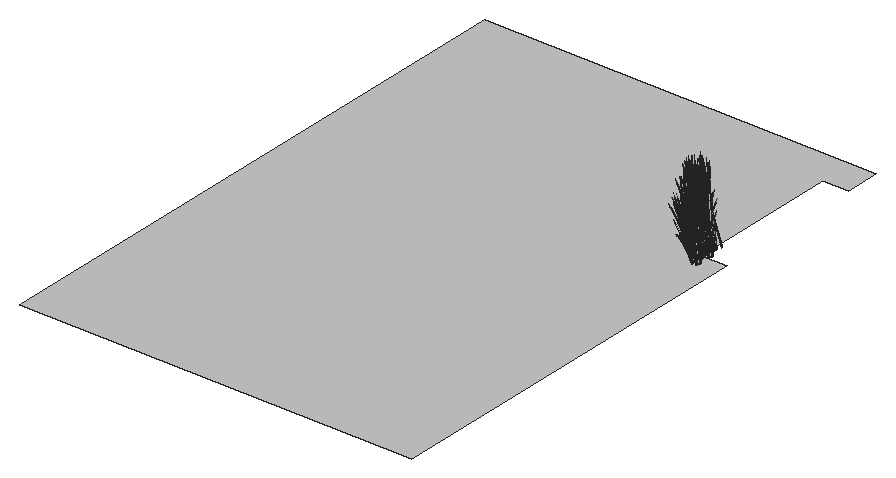
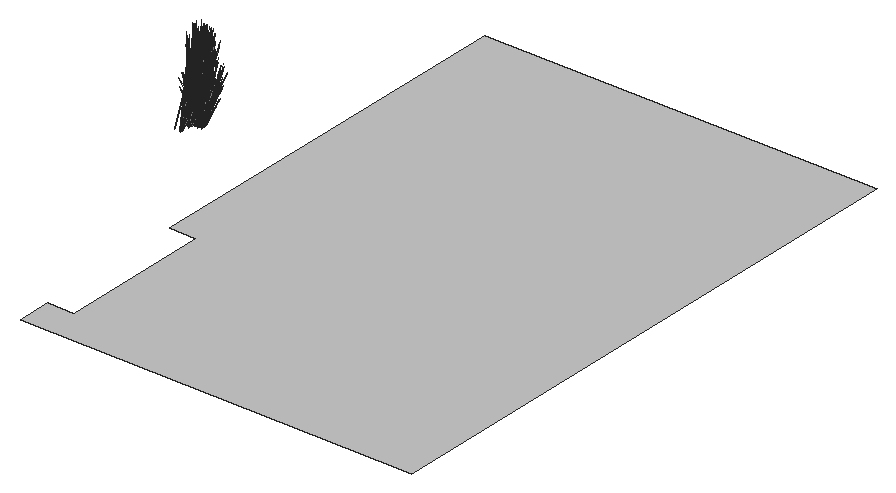
# SketchUp Ruby script. Lengths in inches.
U = 1.inch
M = Sketchup.active_model
def pt(a) = Geom::Point3d.new(a.map { |v| v * U })
def face(e, loops, mat)
  f = e.add_face(loops[0].map { |a| pt(a) })
  loops[1..].each { |l| e.add_face(l.map { |a| pt(a) }).erase! }
  f.material = f.back_material = mat if mat
  f
end
# faces: each face lists its corners as indices into pts; further lists are holes
def faces(e, pts, list, mat = nil) = list.each { |f| face(e, (f[0].is_a?(Array) ? f : [f]).map { |l| l.map { |i| pts[i] } }, mat) }
# xy, xz, yz: faces in a plane at the given z, y or x. An outline is a flat list of corners, or four numbers for a rectangle; further outlines are holes
def ring(l) = l.size == 4 ? [[l[0], l[1]], [l[2], l[1]], [l[2], l[3]], [l[0], l[3]]] : l.each_slice(2).to_a
def flat(e, list, mat, &to3) = list.each { |f| face(e, (f[0].is_a?(Array) ? f : [f]).map { |l| ring(l).map { |u, v| to3.(u, v) } }, mat) }
def xy(e, z, list, mat = nil) = flat(e, list, mat) { |x, y| [x, y, z] }
def xz(e, y, list, mat = nil) = flat(e, list, mat) { |x, z| [x, y, z] }
def yz(e, x, list, mat = nil) = flat(e, list, mat) { |y, z| [x, y, z] }
def lines(e, pts, list) = list.each { |a, b| e.add_line(pt(pts[a]), pt(pts[b])) }
# prism: a flat outline (further loops are holes) pulled along v
def prism(e, loops, v, mat = nil)
  f = face(e, loops, mat); d = Geom::Vector3d.new(v.map { |x| x * U })
  f.pushpull(f.normal.samedirection?(d) ? d.length : -d.length)
end
def box(e, o, s, mat = nil) = prism(e, [[o, [o[0] + s[0], o[1], o[2]], [o[0] + s[0], o[1] + s[1], o[2]], [o[0], o[1] + s[1], o[2]]]], [0, 0, s[2]], mat)
def at(x, y, z, deg = 0) = Geom::Transformation.translation(pt([x, y, z])) * Geom::Transformation.rotation(ORIGIN, Z_AXIS, deg.degrees)
def axes(o, x, y, z) = Geom::Transformation.new([*x, 0, *y, 0, *z, 0, *pt(o).to_a, 1])
def part(name) = M.definitions.add(name)
# library, detail: a bought-in or finely detailed component or shape, given as its bounding box
def library(name, o, s) = part(name).tap { |d| box(d.entities, o, s) }
def detail(e, o, s) = box(e.add_group.entities, o, s)
def put(e, d, t, mat = nil) = e.add_instance(d, t).tap { |i| i.material = mat if mat }
def group(e, t, mat = nil) = e.add_group.tap { |g| g.transformation = t; g.material = mat if mat }.entities
root = M.entities
M.materials.add("LightPink_Translucent").color = [144, 107, 117]
M.materials["LightPink_Translucent"].alpha = 0.75
M.materials.add("[_0053_Ivory_]").color = [200, 200, 200]
c1 = part("blade")
p = [[2.15,0.21,22],[0,0.17,0],[0.09,0.45,0],[2.18,0.31,22],[2.29,0.31,22],[0.38,0.45,0],
  [2.48,0.24,33],[2.49,0.24,33],[2.48,0.22,33]]
faces(c1.entities,p,[[0,1,2,3],[4,5,2,3],[6,3,4,7],[8,0,3,6]])
c2 = part("seeds")
p = [[0.3,-0.1,1.38],[-0.01,-0.03,1.59],[-0.01,-0.03,0.03],[0.14,-0.07,-0.07],[0.29,-0.03,3],[0.15,0.01,3.11]]
faces(c2.entities,p,[[0,1,2,3],[1,0,4,5]],"LightPink_Translucent")
c3 = part("blade with seeds")
put(c3.entities,c1,at(0,0,0))
put(c3.entities,c2,axes([2.4,0.25,30.99],[1.5799,-0.05474,1.17369],[-0.12525,1.92788,0.29478],[-0.07173,-0.02425,1.56792]))
xy(root,0,[[377.51,94.15,377.51,503.15,653.51,503.15,653.51,479.15,635.1,479.15,635.1,371.15,653.51,371.15,653.51,94.15]],"[_0053_Ivory_]")
put(root,c3,axes([670.81,318.54,37.53],[0.25192,-0.01424,1.71376],[-0.16712,0.61729,0.13857],[-0.35901,-0.03818,0.73262]),"[_0053_Ivory_]")
put(root,c3,axes([670.91,319.625,37.53],[0.21074,-0.13302,1.71376],[0.17741,0.61464,0.13857],[-0.33083,0.13891,0.73262]),"[_0053_Ivory_]")
put(root,c3,axes([670.25,320.67,36.24],[0.21107,0.05162,1.43002],[0.13604,0.52729,-0.30754],[-0.28671,0.0987,0.61141]),"[_0053_Ivory_]")
put(root,c3,axes([672.12,318.99,37],[0.17264,-0.09097,1.77064],[0.05953,0.63516,0.13857],[-0.37394,0.08428,0.63284]),"[_0053_Ivory_]")
put(root,c3,axes([671.56,317.97,38.63],[-0.60713,-0.01514,-0.71045],[0.04078,-0.63759,0.08574],[-0.25721,-0.06729,1.00501]),"[_0053_Ivory_]")
put(root,c3,axes([671.07,318.12,36.24],[0.11858,0.17508,1.43002],[-0.27325,0.4759,-0.30754],[-0.28057,-0.11375,0.61141]),"[_0053_Ivory_]")
put(root,c3,axes([670.58,319.07,38.18],[-0.50475,-0.17543,-0.35414],[0.14722,-0.5118,0.4572],[-0.20322,0.04693,0.87481]),"[_0053_Ivory_]")
put(root,c3,axes([671.28,317.55,37.53],[0.2256,0.10835,1.71376],[-0.46687,0.45453,0.13857],[-0.29098,-0.20505,0.73262]),"[_0053_Ivory_]")
put(root,c3,axes([670.93,319.33,38.33],[-0.16454,0.57202,-0.51099],[-0.56413,-0.19607,-0.3958],[-0.22713,0.05245,0.97773]),"[_0053_Ivory_]")
put(root,c3,axes([671.36,318.1,38.33],[-0.44101,0.41656,-0.51099],[-0.38623,-0.44004,-0.3958],[-0.22407,-0.06338,0.97773]),"[_0053_Ivory_]")
put(root,c3,axes([670.65,319.3,35.15],[0.0154,0.09911,1.76342],[-0.31051,0.51756,-0.26939],[-0.22056,-0.02609,0.30037]),"[_0053_Ivory_]")
put(root,c3,axes([669.8125,321.78,36.42],[0.25312,-0.28501,1.1486],[0.09988,0.45119,0.84392],[-0.18292,0.08079,0.25299]),"[_0053_Ivory_]")
put(root,c3,axes([671.19,317.7,38.18],[-0.34557,-0.39372,-0.35414],[0.39459,-0.37271,0.4572],[-0.20048,-0.05671,0.87481]),"[_0053_Ivory_]")
put(root,c3,axes([671.68,320.04,37.53],[0.1517,-0.19322,1.71376],[0.38303,0.52154,0.13857],[-0.26271,0.23751,0.73262]),"[_0053_Ivory_]")
put(root,c3,axes([670.77,320.55,38.18],[-0.52868,0.08987,-0.35414],[-0.1396,-0.51376,0.4572],[-0.1515,0.13799,0.87481]),"[_0053_Ivory_]")
put(root,c3,axes([670.48,322.07,35.15],[0.08147,0.06283,1.76342],[0.13814,0.58211,-0.26939],[-0.18056,0.12413,0.30037]),"[_0053_Ivory_]")
put(root,c3,axes([670.36,318.65,36.42],[0.38775,-0.045,1.1486],[-0.24596,0.39648,0.84392],[-0.19161,-0.05948,0.25299]),"[_0053_Ivory_]")
put(root,c3,axes([671.57,320.52,37.53],[0.11309,-0.21615,1.71376],[0.47441,0.44731,0.13857],[-0.21402,0.27879,0.73262]),"[_0053_Ivory_]")
put(root,c3,axes([671.2,320.61,38.33],[0.15602,0.5742,-0.51099],[-0.59087,0.10045,-0.3958],[-0.16933,0.15423,0.97773]),"[_0053_Ivory_]")
put(root,c3,axes([672.68,320.19,35.71],[-0.63179,-0.1031,-0.62353],[0.13332,-0.63596,-0.16365],[-0.18854,-0.07706,1.37633]),"[_0053_Ivory_]")
put(root,c3,axes([672.61,317.22,38.63],[-0.51789,-0.30395,-0.71045],[0.36805,-0.53263,0.08574],[-0.18764,-0.18149,1.00501]),"[_0053_Ivory_]")
put(root,c3,axes([672.37,317.23,38.33],[-0.59932,0.14948,-0.51099],[-0.10484,-0.56611,-0.3958],[-0.16097,-0.16223,0.97773]),"[_0053_Ivory_]")
put(root,c3,axes([671.85,321.4,35.67],[-0.56842,-0.31443,-0.49651],[0.33976,-0.56381,0],[-0.12946,-0.07161,1.57504]),"[_0053_Ivory_]")
put(root,c3,axes([671.6,316.71,35.15],[-0.05883,0.08284,1.76342],[-0.59454,0.17861,-0.26939],[-0.14363,-0.16248,0.30037]),"[_0053_Ivory_]")
put(root,c3,axes([672.19,321.78,36.03],[-0.37973,0.63014,0],[-0.6353,-0.35142,-0.51607],[-0.14469,-0.08004,1.63711]),"[_0053_Ivory_]")
put(root,c3,axes([671.5,322.69,36.24],[0.19166,-0.0992,1.43002],[0.4732,0.29912,-0.30754],[-0.14084,0.25882,0.61141]),"[_0053_Ivory_]")
put(root,c3,axes([671.23,317.03,35.78],[-0.1752,0.51349,-0.03893],[-0.53924,-0.15795,-0.17649],[-0.08187,-0.08399,0.58215]),"[_0053_Ivory_]")
put(root,c3,axes([672.03,316.39,36.24],[-0.03678,0.20572,1.43002],[-0.53767,0.17221,-0.30754],[-0.12568,-0.26589,0.61141]),"[_0053_Ivory_]")
put(root,c3,axes([672.21,316.92,37.53],[0.13883,0.2019,1.71376],[-0.64153,0.16998,0.13857],[-0.14499,-0.31697,0.73262]),"[_0053_Ivory_]")
put(root,c3,axes([673.39,320.29,36.32],[-0.61322,0.4175,-0.29095],[-0.40778,-0.58992,-0.50002],[-0.1513,-0.05991,1.59708]),"[_0053_Ivory_]")
put(root,c3,axes([672.43,316.8125,38.18],[-0.0938,-0.50652,-0.35414],[0.53623,-0.13375,0.4572],[-0.14403,-0.14515,0.87481]),"[_0053_Ivory_]")
put(root,c3,axes([670.94,319.38,36.03],[-0.75945,0,0],[0,-0.70283,-0.51607],[0,-0.16007,1.63711]),"[_0053_Ivory_]")
put(root,c3,axes([672.01,321.16,35.68],[-0.14267,-0.54795,-0.30978],[0.56663,-0.1556,0.30978],[-0.11423,-0.06319,1.38974]),"[_0053_Ivory_]")
put(root,c3,axes([671.7,321.74,38.18],[-0.41095,0.33109,-0.35414],[-0.38901,-0.37805,0.4572],[-0.05919,0.19208,0.87481]),"[_0053_Ivory_]")
put(root,c3,axes([673.8,320.74,35.71],[-0.40909,0.47266,-0.62353],[-0.50819,-0.4286,-0.16365],[-0.16393,0.11791,1.37633]),"[_0053_Ivory_]")
put(root,c3,axes([671.53,319.19,35.98],[-0.56493,0.5287,0.30756],[-0.56528,-0.52313,-0.36492],[-0.01973,-0.15014,1.64885]),"[_0053_Ivory_]")
put(root,c3,axes([673.85,320.65,36.98],[0.52485,0.25358,1.51261],[-0.51417,0.54629,0.59816],[-0.23031,-0.32378,1.26806]),"[_0053_Ivory_]")
put(root,c3,axes([671.85,316.06,36.42],[0.31682,0.21887,1.1486],[-0.4614,0.13157,0.84392],[-0.09872,-0.16821,0.25299]),"[_0053_Ivory_]")
put(root,c3,axes([674.08,320.48,36.12],[-0.59306,-0.50614,-0.25192],[0.49904,-0.56836,0.5513],[-0.1597,0.05921,1.68216]),"[_0053_Ivory_]")
put(root,c3,axes([673,319.99,35.86],[-0.36485,-0.52782,-0.44739],[0.55265,-0.37168,0.21531],[-0.11807,-0.06531,1.43643]),"[_0053_Ivory_]")
put(root,c3,axes([671.97,321.39,38.99],[-0.0158,0.58168,-0.7886],[-0.66548,-0.03907,0.09517],[-0.07023,0.24643,1.11556]),"[_0053_Ivory_]")
put(root,c3,axes([671.96,323.02,36.42],[-0.01572,-0.37392,1.1486],[0.39276,0.26669,0.84392],[-0.07724,0.17822,0.25299]),"[_0053_Ivory_]")
put(root,c3,axes([673.78,320.37,35.86],[-0.65953,0.03882,-0.44739],[-0.05964,-0.64439,0.21531],[-0.11807,0.06531,1.43643]),"[_0053_Ivory_]")
put(root,c3,axes([677.08,321.61,37.53],[0.25192,-0.01424,1.71376],[-0.16712,0.61729,0.13857],[-0.35901,-0.03818,0.73262]),"[_0053_Ivory_]")
put(root,c3,axes([672.52,321.45,36.13],[0.56842,0.31443,0.49651],[-0.33976,0.56381,0],[-0.12946,-0.07161,1.57504]),"[_0053_Ivory_]")
put(root,c3,axes([671.75,322.21,37.02],[0.01334,-0.32463,1.54345],[0.60018,0.17147,0.21329],[-0.052,0.34598,0.72882]),"[_0053_Ivory_]")
put(root,c3,axes([673.06,320.3,36.09],[0.16098,-0.74515,-0.23429],[0.76326,0.12989,0.51271],[-0.13337,-0.1029,1.5644]),"[_0053_Ivory_]")
put(root,c3,axes([673.34,320.47,36.27],[-0.11717,0.56122,0.1448],[-0.57245,-0.09742,-0.41347],[-0.10418,-0.05763,1.26744]),"[_0053_Ivory_]")
put(root,c3,axes([674.47,322.03,35.67],[-0.56842,0.31443,-0.49651],[-0.33976,-0.56381,0],[-0.12946,0.07161,1.57504]),"[_0053_Ivory_]")
put(root,c3,axes([671.11,318.9,35.67],[0,-0.62885,-0.49651],[0.67951,0,0],[0,-0.14322,1.57504]),"[_0053_Ivory_]")
put(root,c3,axes([671.4,319.48,36.13],[0,0.62885,0.49651],[-0.67951,0,0],[0,-0.14322,1.57504]),"[_0053_Ivory_]")
put(root,c3,axes([674.51,321.87,35.85],[-0.37499,-0.63235,-0.05142],[0.6353,-0.35142,0.51607],[-0.15655,0.0602,1.6363]),"[_0053_Ivory_]")
put(root,c3,axes([672.11,321.58,38.66],[0.43478,0.42253,-0.5672],[-0.45929,0.37004,-0.43934],[-0.06615,0.21468,1.08528]),"[_0053_Ivory_]")
put(root,c3,axes([674.34,321.79,35.68],[-0.56663,-0.1556,-0.30978],[0.14267,-0.54795,0.30978],[-0.11423,0.06319,1.38974]),"[_0053_Ivory_]")
put(root,c3,axes([677.1875,312.1,37.53],[0.21074,-0.13302,1.71376],[0.17741,0.61464,0.13857],[-0.33083,0.13891,0.73262]),"[_0053_Ivory_]")
put(root,c3,axes([677.1875,322.69,37.53],[0.21074,-0.13302,1.71376],[0.17741,0.61464,0.13857],[-0.33083,0.13891,0.73262]),"[_0053_Ivory_]")
put(root,c3,axes([672.89,319.63,36.32],[-0.68399,-0.30005,-0.29095],[0.32934,-0.63331,-0.50002],[-0.0215,-0.15549,1.59708]),"[_0053_Ivory_]")
put(root,c3,axes([674.67,319.44,36.5],[-0.01659,-0.59209,1.41272],[0.75089,0.15348,0.59816],[-0.1776,0.32398,1.3335]),"[_0053_Ivory_]")
put(root,c3,axes([676.53,313.15,36.24],[0.21107,0.05162,1.43002],[0.13604,0.52729,-0.30754],[-0.28671,0.0987,0.61141]),"[_0053_Ivory_]")
put(root,c3,axes([676.53,323.74,36.24],[0.21107,0.05162,1.43002],[0.13604,0.52729,-0.30754],[-0.28671,0.0987,0.61141]),"[_0053_Ivory_]")
put(root,c3,axes([671.63,322.21,36.48],[0.55175,-0.11136,0.06507],[0.12684,0.44864,-0.86304],[-0.03498,0.22711,0.7736]),"[_0053_Ivory_]")
put(root,c3,axes([674.24,320.2,36.32],[0.07077,0.71755,-0.29095],[-0.73712,0.04339,-0.50002],[-0.1298,0.09558,1.59708]),"[_0053_Ivory_]")
put(root,c3,axes([672.58,318.99,35.75],[-0.24943,-0.64486,-0.69835],[0.71849,-0.23224,-0.18329],[-0.02757,-0.21836,1.54149]),"[_0053_Ivory_]")
put(root,c3,axes([678.4,311.46,37],[0.17264,-0.09097,1.77064],[0.05953,0.63516,0.13857],[-0.37394,0.08428,0.63284]),"[_0053_Ivory_]")
put(root,c3,axes([678.4,322.05,37],[0.17264,-0.09097,1.77064],[0.05953,0.63516,0.13857],[-0.37394,0.08428,0.63284]),"[_0053_Ivory_]")
put(root,c3,axes([673.7,316.97,38.33],[-0.59704,-0.15764,-0.51099],[0.20464,-0.54049,-0.3958],[-0.05475,-0.21761,0.97773]),"[_0053_Ivory_]")
put(root,c3,axes([672.6,320.97,37.53],[-0.01487,-0.24136,1.71376],[0.64429,0.16012,0.13857],[-0.03985,0.34396,0.73262]),"[_0053_Ivory_]")
put(root,c3,axes([671.4,318.91,35.68],[0.42396,-0.39235,-0.30978],[0.42396,0.39235,0.30978],[0,-0.12637,1.38974]),"[_0053_Ivory_]")
put(root,c3,axes([673.32,316.38,35.78],[-0.4197,0.36076,-0.03893],[-0.38456,-0.39511,-0.17649],[-0.02707,-0.11196,0.58215]),"[_0053_Ivory_]")
put(root,c3,axes([673.15,319.9375,36.01],[0.76764,0.13249,0.45755],[-0.15622,0.74829,0.17955],[-0.11218,-0.07226,1.58856]),"[_0053_Ivory_]")
put(root,c3,axes([677.83,321.03,38.63],[-0.60713,-0.01514,-0.71045],[0.04078,-0.63759,0.08574],[-0.25721,-0.06729,1.00501]),"[_0053_Ivory_]")
put(root,c3,axes([677.35,321.19,36.24],[0.11858,0.17508,1.43002],[-0.27325,0.4759,-0.30754],[-0.28057,-0.11375,0.61141]),"[_0053_Ivory_]")
put(root,c3,axes([672.95,319.8,36.37],[-0.29468,0.56664,0.44739],[-0.61229,-0.27271,-0.21531],[0,-0.13062,1.43643]),"[_0053_Ivory_]")
put(root,c3,axes([673.92,317.07,38.63],[-0.28988,-0.51132,-0.71045],[0.59671,-0.28496,0.08574],[-0.06778,-0.24706,1.00501]),"[_0053_Ivory_]")
put(root,c3,axes([676.86,311.55,38.18],[-0.50475,-0.17543,-0.35414],[0.14722,-0.5118,0.4572],[-0.20322,0.04693,0.87481]),"[_0053_Ivory_]")
put(root,c3,axes([676.86,322.14,38.18],[-0.50475,-0.17543,-0.35414],[0.14722,-0.5118,0.4572],[-0.20322,0.04693,0.87481]),"[_0053_Ivory_]")
put(root,c3,axes([677.56,320.62,37.53],[0.2256,0.10835,1.71376],[-0.46687,0.45453,0.13857],[-0.29098,-0.20505,0.73262]),"[_0053_Ivory_]")
put(root,c3,axes([677.56,330.76,37.53],[0.2256,0.10835,1.71376],[-0.46687,0.45453,0.13857],[-0.29098,-0.20505,0.73262]),"[_0053_Ivory_]")
put(root,c3,axes([672.73,321.13,36.13],[0.65264,-0.16691,0.17642],[0.16115,0.62115,0.35086],[-0.05821,-0.0905,1.60407]),"[_0053_Ivory_]")
put(root,c3,axes([677.21,311.81,38.33],[-0.16454,0.57202,-0.51099],[-0.56413,-0.19607,-0.3958],[-0.22713,0.05245,0.97773]),"[_0053_Ivory_]")
put(root,c3,axes([677.21,322.4,38.33],[-0.16454,0.57202,-0.51099],[-0.56413,-0.19607,-0.3958],[-0.22713,0.05245,0.97773]),"[_0053_Ivory_]")
put(root,c3,axes([673.57,321.23,35.85],[-0.61229,-0.28233,0],[0.29468,-0.58663,0],[0,0,1.62707]),"[_0053_Ivory_]")
put(root,c3,axes([674.99,321.9375,36.03],[0.37973,0.63014,0],[-0.6353,0.35142,-0.51607],[-0.14469,0.08004,1.63711]),"[_0053_Ivory_]")
put(root,c3,axes([677.63,321.16,38.33],[-0.44101,0.41656,-0.51099],[-0.38623,-0.44004,-0.3958],[-0.22407,-0.06338,0.97773]),"[_0053_Ivory_]")
put(root,c3,axes([676.92,311.77,35.15],[0.0154,0.09911,1.76342],[-0.31051,0.51756,-0.26939],[-0.22056,-0.02609,0.30037]),"[_0053_Ivory_]")
put(root,c3,axes([676.92,322.36,35.15],[0.0154,0.09911,1.76342],[-0.31051,0.51756,-0.26939],[-0.22056,-0.02609,0.30037]),"[_0053_Ivory_]")
put(root,c3,axes([674.68,321.17,36.13],[0.17545,-0.62497,0.17642],[0.64204,0.17686,0.35086],[-0.11091,0.00304,1.60407]),"[_0053_Ivory_]")
put(root,c3,axes([674.38,320.34,36.27],[0.44871,0.37783,0.1448],[-0.37428,0.42627,-0.41347],[-0.10418,0.05763,1.26744]),"[_0053_Ivory_]")
put(root,c3,axes([676.09,314.25,36.42],[0.25312,-0.28501,1.1486],[0.09988,0.45119,0.84392],[-0.18292,0.08079,0.25299]),"[_0053_Ivory_]")
put(root,c3,axes([676.09,324.85,36.42],[0.25312,-0.28501,1.1486],[0.09988,0.45119,0.84392],[-0.18292,0.08079,0.25299]),"[_0053_Ivory_]")
put(root,c3,axes([674.22,319.87,35.95],[-0.56493,-0.54126,-0.06131],[0.56528,-0.54159,0],[-0.01973,-0.0189,1.75571]),"[_0053_Ivory_]")
put(root,c3,axes([674.37,320.06,36.37],[0.65953,-0.03882,0.44739],[0.05964,0.64439,-0.21531],[-0.11807,0.06531,1.43643]),"[_0053_Ivory_]")
put(root,c3,axes([674.53,321.54,35.98],[0.76036,0.2044,0.30756],[-0.19023,0.7306,-0.36492],[-0.12585,0.09144,1.64885]),"[_0053_Ivory_]")
put(root,c3,axes([673.42,315.9375,35.15],[-0.10187,0.02266,1.76342],[-0.56336,-0.25503,-0.26939],[0.00945,-0.21273,0.30037]),"[_0053_Ivory_]")
put(root,c3,axes([674.86,321.5,36.13],[0.56842,-0.31443,0.49651],[0.33976,0.56381,0],[-0.12946,0.07161,1.57504]),"[_0053_Ivory_]")
put(root,c3,axes([677.47,320.77,38.18],[-0.34557,-0.39372,-0.35414],[0.39459,-0.37271,0.4572],[-0.20048,-0.05671,0.87481]),"[_0053_Ivory_]")
put(root,c3,axes([677.47,330.91,38.18],[-0.34557,-0.39372,-0.35414],[0.39459,-0.37271,0.4572],[-0.20048,-0.05671,0.87481]),"[_0053_Ivory_]")
put(root,c3,axes([673.98,316.64,38.18],[0.1831,-0.48359,-0.35414],[0.53419,0.14105,0.4572],[-0.04898,-0.1947,0.87481]),"[_0053_Ivory_]")
put(root,c3,axes([673.08,319.25,36.01],[0.26406,0.70318,0.45755],[-0.7545,0.24452,0.17955],[0.00922,-0.12921,1.58856]),"[_0053_Ivory_]")
put(root,c3,axes([677.96,312.52,37.53],[0.1517,-0.19322,1.71376],[0.38303,0.52154,0.13857],[-0.26271,0.23751,0.73262]),"[_0053_Ivory_]")
put(root,c3,axes([677.96,323.11,37.53],[0.1517,-0.19322,1.71376],[0.38303,0.52154,0.13857],[-0.26271,0.23751,0.73262]),"[_0053_Ivory_]")
put(root,c3,axes([677.04,313.02,38.18],[-0.52868,0.08987,-0.35414],[-0.1396,-0.51376,0.4572],[-0.1515,0.13799,0.87481]),"[_0053_Ivory_]")
put(root,c3,axes([677.04,323.61,38.18],[-0.52868,0.08987,-0.35414],[-0.1396,-0.51376,0.4572],[-0.1515,0.13799,0.87481]),"[_0053_Ivory_]")
put(root,c3,axes([672.96,319.16,35.86],[0.29468,-0.56664,-0.44739],[0.61229,0.27271,0.21531],[0,-0.13062,1.43643]),"[_0053_Ivory_]")
put(root,c3,axes([673.71,320.98,35.86],[-0.19817,-0.54216,0],[0.56587,-0.18986,0],[0,0,1.54371]),"[_0053_Ivory_]")
put(root,c3,axes([672.99,322.13,35.15],[0.09829,-0.03422,1.76342],[0.59126,0.18834,-0.26939],[0.01729,0.21228,0.30037]),"[_0053_Ivory_]")
put(root,c3,axes([676.76,314.55,35.15],[0.08147,0.06283,1.76342],[0.13814,0.58211,-0.26939],[-0.18056,0.12413,0.30037]),"[_0053_Ivory_]")
put(root,c3,axes([676.76,325.14,35.15],[0.08147,0.06283,1.76342],[0.13814,0.58211,-0.26939],[-0.18056,0.12413,0.30037]),"[_0053_Ivory_]")
put(root,c3,axes([673.125,322.32,38.18],[-0.1831,0.48359,-0.35414],[-0.53419,-0.14105,0.4572],[0.04898,0.1947,0.87481]),"[_0053_Ivory_]")
put(root,c3,axes([676.64,321.72,36.42],[0.38775,-0.045,1.1486],[-0.24596,0.39648,0.84392],[-0.19161,-0.05948,0.25299]),"[_0053_Ivory_]")
put(root,c3,axes([674.51,319.92,35.86],[-0.29468,0.56664,-0.44739],[-0.61229,-0.27271,0.21531],[0,0.13062,1.43643]),"[_0053_Ivory_]")
put(root,c3,axes([675.68,319.57,36.13],[-0.47719,-0.45806,0.17642],[0.48088,-0.44429,0.35086],[-0.0527,0.09355,1.60407]),"[_0053_Ivory_]")
put(root,c3,axes([674.03,319.31,35.86],[0,-0.72763,0],[0.75945,0,0],[0,0,1.79456]),"[_0053_Ivory_]")
put(root,c3,axes([677.84,312.99,37.53],[0.11309,-0.21615,1.71376],[0.47441,0.44731,0.13857],[-0.21402,0.27879,0.73262]),"[_0053_Ivory_]")
put(root,c3,axes([677.84,323.59,37.53],[0.11309,-0.21615,1.71376],[0.47441,0.44731,0.13857],[-0.21402,0.27879,0.73262]),"[_0053_Ivory_]")
put(root,c3,axes([673.32,319.4375,36.09],[0.68433,0.30479,0.24065],[-0.32934,0.63331,0.50002],[0,-0.14599,1.60543]),"[_0053_Ivory_]")
put(root,c3,axes([674.41,319.6,35.95],[0,0.72727,-0.05637],[-0.75945,0,0],[0,0.02286,1.79368]),"[_0053_Ivory_]")
put(root,c3,axes([673.1,319.01,36.37],[-0.65953,0.03882,0.44739],[-0.05964,-0.64439,-0.21531],[0.11807,-0.06531,1.43643]),"[_0053_Ivory_]")
put(root,c3,axes([672.8,317.91,36.13],[-0.17545,0.62497,0.17642],[-0.64204,-0.17686,0.35086],[0.11091,-0.00304,1.60407]),"[_0053_Ivory_]")
put(root,c3,axes([674.05,321,35.94],[0.26406,0.72244,-0.06012],[-0.7545,0.25315,0],[0.00922,0.02523,1.72173]),"[_0053_Ivory_]")
put(root,c3,axes([677.48,313.08,38.33],[0.15602,0.5742,-0.51099],[-0.59087,0.10045,-0.3958],[-0.16933,0.15423,0.97773]),"[_0053_Ivory_]")
put(root,c3,axes([677.48,323.67,38.33],[0.15602,0.5742,-0.51099],[-0.59087,0.10045,-0.3958],[-0.16933,0.15423,0.97773]),"[_0053_Ivory_]")
put(root,c3,axes([678.95,312.67,35.71],[-0.63179,-0.1031,-0.62353],[0.13332,-0.63596,-0.16365],[-0.18854,-0.07706,1.37633]),"[_0053_Ivory_]")
put(root,c3,axes([678.95,323.26,35.71],[-0.63179,-0.1031,-0.62353],[0.13332,-0.63596,-0.16365],[-0.18854,-0.07706,1.37633]),"[_0053_Ivory_]")
put(root,c3,axes([672.48,317.14,36.03],[-0.37973,-0.63014,0],[0.6353,-0.35142,-0.51607],[0.14469,-0.08004,1.63711]),"[_0053_Ivory_]")
put(root,c3,axes([673.18,321.89,38.63],[0.28988,0.51132,-0.71045],[-0.59671,0.28496,0.08574],[0.06778,0.24706,1.00501]),"[_0053_Ivory_]")
put(root,c3,axes([676.23,320.06,35.85],[-0.75908,-0.00503,-0.04976],[0,-0.70283,0.49943],[-0.02386,0.16,1.58352]),"[_0053_Ivory_]")
put(root,c3,axes([674.74,317.94,36.13],[-0.65264,0.16691,0.17642],[-0.16115,-0.62115,0.35086],[0.05821,0.0905,1.60407]),"[_0053_Ivory_]")
put(root,c3,axes([678.89,320.28,38.63],[-0.51789,-0.30395,-0.71045],[0.36805,-0.53263,0.08574],[-0.18764,-0.18149,1.00501]),"[_0053_Ivory_]")
put(root,c3,axes([678.89,330.42,38.63],[-0.51789,-0.30395,-0.71045],[0.36805,-0.53263,0.08574],[-0.18764,-0.18149,1.00501]),"[_0053_Ivory_]")
put(root,c3,axes([678.65,320.3,38.33],[-0.59932,0.14948,-0.51099],[-0.10484,-0.56611,-0.3958],[-0.16097,-0.16223,0.97773]),"[_0053_Ivory_]")
put(root,c3,axes([678.65,330.4375,38.33],[-0.59932,0.14948,-0.51099],[-0.10484,-0.56611,-0.3958],[-0.16097,-0.16223,0.97773]),"[_0053_Ivory_]")
put(root,c3,axes([674.07,315.61,36.42],[0.07791,0.3667,1.1486],[-0.43222,-0.2031,0.84392],[0.04651,-0.18776,0.25299]),"[_0053_Ivory_]")
put(root,c3,axes([673.67,318.85,36.01],[-0.50358,0.57069,0.45755],[-0.59827,-0.50377,0.17955],[0.1214,-0.05695,1.58856]),"[_0053_Ivory_]")
put(root,c3,axes([678.125,313.875,35.67],[-0.56842,-0.31443,-0.49651],[0.33976,-0.56381,0],[-0.12946,-0.07161,1.57504]),"[_0053_Ivory_]")
put(root,c3,axes([678.125,324.47,35.67],[-0.56842,-0.31443,-0.49651],[0.33976,-0.56381,0],[-0.12946,-0.07161,1.57504]),"[_0053_Ivory_]")
put(root,c3,axes([674.53,319.75,35.87],[0.42396,0.40619,0],[-0.42396,0.40619,0],[0,0,1.69266]),"[_0053_Ivory_]")
put(root,c3,axes([677.875,319.78,35.15],[-0.05883,0.08284,1.76342],[-0.59454,0.17861,-0.26939],[-0.14363,-0.16248,0.30037]),"[_0053_Ivory_]")
put(root,c3,axes([677.875,329.92,35.15],[-0.05883,0.08284,1.76342],[-0.59454,0.17861,-0.26939],[-0.14363,-0.16248,0.30037]),"[_0053_Ivory_]")
put(root,c3,axes([674.52,319.27,36.37],[0.29468,-0.56664,0.44739],[0.61229,0.27271,-0.21531],[0,0.13062,1.43643]),"[_0053_Ivory_]")
put(root,c3,axes([674.27,321.24,35.86],[0.61229,0.28233,0],[-0.29468,0.58663,0],[0,0,1.74954]),"[_0053_Ivory_]")
put(root,c3,axes([678.47,314.25,36.03],[-0.37973,0.63014,0],[-0.6353,-0.35142,-0.51607],[-0.14469,-0.08004,1.63711]),"[_0053_Ivory_]")
put(root,c3,axes([678.47,324.85,36.03],[-0.37973,0.63014,0],[-0.6353,-0.35142,-0.51607],[-0.14469,-0.08004,1.63711]),"[_0053_Ivory_]")
put(root,c3,axes([673.4,321.99,38.33],[0.59704,0.15764,-0.51099],[-0.20464,0.54049,-0.3958],[0.05475,0.21761,0.97773]),"[_0053_Ivory_]")
put(root,c3,axes([674.33,319.14,36.03],[-0.76764,-0.13249,0.49198],[0.15622,-0.74829,0.19306],[0.11218,0.07226,1.70813]),"[_0053_Ivory_]")
put(root,c3,axes([676.07,320.16,35.68],[-0.42396,0.39235,-0.30978],[-0.42396,-0.39235,0.30978],[0,0.12637,1.38974]),"[_0053_Ivory_]")
put(root,c3,axes([674.86,320.09,35.75],[0.2227,0.57576,-0.69212],[-0.64151,0.20736,-0.18165],[0.02462,0.19497,1.52773]),"[_0053_Ivory_]")
put(root,c3,axes([674.55,319.47,35.86],[0.67951,0,0],[0,0.65103,0],[0,0,1.78407]),"[_0053_Ivory_]")
put(root,c3,axes([677.78,315.17,36.24],[0.19166,-0.0992,1.43002],[0.4732,0.29912,-0.30754],[-0.14084,0.25882,0.61141]),"[_0053_Ivory_]")
put(root,c3,axes([673.89,318.75,36.37],[-0.36485,-0.52782,0.44739],[0.55265,-0.37168,-0.21531],[0.11807,0.06531,1.43643]),"[_0053_Ivory_]")
put(root,c3,axes([673.23,318.875,36.32],[-0.07077,-0.71755,-0.29095],[0.73712,-0.04339,-0.50002],[0.1298,-0.09558,1.59708]),"[_0053_Ivory_]")
put(root,c3,axes([674.78,319.4,36.27],[0.56587,-0.18339,0.1448],[0.19817,0.52368,-0.41347],[0,0.11525,1.26744]),"[_0053_Ivory_]")
put(root,c3,axes([674.99,317.38,38.33],[-0.43478,-0.42253,-0.51099],[0.45929,-0.37004,-0.3958],[0.06615,-0.21468,0.97773]),"[_0053_Ivory_]")
put(root,c3,axes([677.51,320.1,35.78],[-0.1752,0.51349,-0.03893],[-0.53924,-0.15795,-0.17649],[-0.08187,-0.08399,0.58215]),"[_0053_Ivory_]")
put(root,c3,axes([677.51,330.24,35.78],[-0.1752,0.51349,-0.03893],[-0.53924,-0.15795,-0.17649],[-0.08187,-0.08399,0.58215]),"[_0053_Ivory_]")
put(root,c3,axes([678.3125,319.45,36.24],[-0.03678,0.20572,1.43002],[-0.53767,0.17221,-0.30754],[-0.12568,-0.26589,0.61141]),"[_0053_Ivory_]")
put(root,c3,axes([678.3125,329.59,36.24],[-0.03678,0.20572,1.43002],[-0.53767,0.17221,-0.30754],[-0.12568,-0.26589,0.61141]),"[_0053_Ivory_]")
put(root,c3,axes([674.59,319.44,36.32],[0.68399,0.30005,-0.29095],[-0.32934,0.63331,-0.50002],[0.0215,0.15549,1.59708]),"[_0053_Ivory_]")
put(root,c3,axes([678.49,319.99,37.53],[0.13883,0.2019,1.71376],[-0.64153,0.16998,0.13857],[-0.14499,-0.31697,0.73262]),"[_0053_Ivory_]")
put(root,c3,axes([678.49,330.13,37.53],[0.13883,0.2019,1.71376],[-0.64153,0.16998,0.13857],[-0.14499,-0.31697,0.73262]),"[_0053_Ivory_]")
put(root,c3,axes([679.67,312.76,36.32],[-0.61322,0.4175,-0.29095],[-0.40778,-0.58992,-0.50002],[-0.1513,-0.05991,1.59708]),"[_0053_Ivory_]")
put(root,c3,axes([679.67,323.36,36.32],[-0.61322,0.4175,-0.29095],[-0.40778,-0.58992,-0.50002],[-0.1513,-0.05991,1.59708]),"[_0053_Ivory_]")
put(root,c3,axes([673.13,317.29,35.68],[0.56663,0.1556,-0.30978],[-0.14267,0.54795,0.30978],[0.11423,-0.06319,1.38974]),"[_0053_Ivory_]")
put(root,c3,axes([678.71,319.88,38.18],[-0.0938,-0.50652,-0.35414],[0.53623,-0.13375,0.4572],[-0.14403,-0.14515,0.87481]),"[_0053_Ivory_]")
put(root,c3,axes([678.71,330.02,38.18],[-0.0938,-0.50652,-0.35414],[0.53623,-0.13375,0.4572],[-0.14403,-0.14515,0.87481]),"[_0053_Ivory_]")
put(root,c3,axes([674.71,316.63,36.24],[-0.17264,0.12729,1.43002],[-0.51703,-0.22279,-0.30754],[0.09584,-0.27707,0.61141]),"[_0053_Ivory_]")
put(root,c3,axes([677.22,322.45,36.03],[-0.75945,0,0],[0,-0.70283,-0.51607],[0,-0.16007,1.63711]),"[_0053_Ivory_]")
put(root,c3,axes([677.22,332.59,36.03],[-0.75945,0,0],[0,-0.70283,-0.51607],[0,-0.16007,1.63711]),"[_0053_Ivory_]")
put(root,c3,axes([678.28,313.64,35.68],[-0.14267,-0.54795,-0.30978],[0.56663,-0.1556,0.30978],[-0.11423,-0.06319,1.38974]),"[_0053_Ivory_]")
put(root,c3,axes([678.28,324.23,35.68],[-0.14267,-0.54795,-0.30978],[0.56663,-0.1556,0.30978],[-0.11423,-0.06319,1.38974]),"[_0053_Ivory_]")
put(root,c3,axes([676.07,319.59,36.13],[0,-0.62885,0.49651],[0.67951,0,0],[0,0.14322,1.57504]),"[_0053_Ivory_]")
put(root,c3,axes([676.36,320.17,35.67],[0,0.62885,-0.49651],[-0.67951,0,0],[0,0.14322,1.57504]),"[_0053_Ivory_]")
put(root,c3,axes([677.97,314.21,38.18],[-0.41095,0.33109,-0.35414],[-0.38901,-0.37805,0.4572],[-0.05919,0.19208,0.87481]),"[_0053_Ivory_]")
put(root,c3,axes([677.97,324.8,38.18],[-0.41095,0.33109,-0.35414],[-0.38901,-0.37805,0.4572],[-0.05919,0.19208,0.87481]),"[_0053_Ivory_]")
put(root,c3,axes([673,317.04,35.67],[0.56842,-0.31443,-0.49651],[0.33976,0.56381,0],[0.12946,-0.07161,1.57504]),"[_0053_Ivory_]")
put(root,c3,axes([673.74,320.875,37.53],[-0.13883,-0.2019,1.71376],[0.64153,-0.16998,0.13857],[0.14499,0.31697,0.73262]),"[_0053_Ivory_]")
put(root,c3,axes([674.14,318.6,36.27],[0.11717,-0.56122,0.1448],[0.57245,0.09742,-0.41347],[0.10418,0.05763,1.26744]),"[_0053_Ivory_]")
put(root,c3,axes([680.08,313.22,35.71],[-0.40909,0.47266,-0.62353],[-0.50819,-0.4286,-0.16365],[-0.16393,0.11791,1.37633]),"[_0053_Ivory_]")
put(root,c3,axes([680.08,323.8125,35.71],[-0.40909,0.47266,-0.62353],[-0.50819,-0.4286,-0.16365],[-0.16393,0.11791,1.37633]),"[_0053_Ivory_]")
put(root,c3,axes([677.8,322.26,35.98],[-0.56493,0.5287,0.30756],[-0.56528,-0.52313,-0.36492],[-0.01973,-0.15014,1.64885]),"[_0053_Ivory_]")
put(root,c3,axes([674.95,317.625,36.13],[-0.56842,-0.31443,0.49651],[0.33976,-0.56381,0],[0.12946,0.07161,1.57504]),"[_0053_Ivory_]")
put(root,c3,axes([675.13,317.57,38.63],[0.0158,-0.58168,-0.71045],[0.66548,0.03907,0.08574],[0.07023,-0.24643,1.00501]),"[_0053_Ivory_]")
put(root,c3,axes([680.13,323.72,36.98],[0.52485,0.25358,1.51261],[-0.51417,0.54629,0.59816],[-0.23031,-0.32378,1.26806]),"[_0053_Ivory_]")
put(root,c3,axes([680.13,333.86,36.98],[0.52485,0.25358,1.51261],[-0.51417,0.54629,0.59816],[-0.23031,-0.32378,1.26806]),"[_0053_Ivory_]")
put(root,c3,axes([674.46,320.91,35.84],[0.63764,-0.21337,-0.19198],[0.22406,0.61462,0.00008],[0.07038,-0.02358,1.73897]),"[_0053_Ivory_]")
put(root,c3,axes([678.125,319.12,36.42],[0.31682,0.21887,1.1486],[-0.4614,0.13157,0.84392],[-0.09872,-0.16821,0.25299]),"[_0053_Ivory_]")
put(root,c3,axes([678.125,329.26,36.42],[0.31682,0.21887,1.1486],[-0.4614,0.13157,0.84392],[-0.09872,-0.16821,0.25299]),"[_0053_Ivory_]")
put(root,c3,axes([680.36,312.95,36.12],[-0.59306,-0.50614,-0.25192],[0.49904,-0.56836,0.5513],[-0.1597,0.05921,1.68216]),"[_0053_Ivory_]")
put(root,c3,axes([680.36,323.55,36.12],[-0.59306,-0.50614,-0.25192],[0.49904,-0.56836,0.5513],[-0.1597,0.05921,1.68216]),"[_0053_Ivory_]")
put(root,c3,axes([679.28,323.06,35.86],[-0.36485,-0.52782,-0.44739],[0.55265,-0.37168,0.21531],[-0.11807,-0.06531,1.43643]),"[_0053_Ivory_]")
put(root,c3,axes([678.25,313.86,38.99],[-0.0158,0.58168,-0.7886],[-0.66548,-0.03907,0.09517],[-0.07023,0.24643,1.11556]),"[_0053_Ivory_]")
put(root,c3,axes([678.24,315.5,36.42],[-0.01572,-0.37392,1.1486],[0.39276,0.26669,0.84392],[-0.07724,0.17822,0.25299]),"[_0053_Ivory_]")
put(root,c3,axes([678.24,326.09,36.42],[-0.01572,-0.37392,1.1486],[0.39276,0.26669,0.84392],[-0.07724,0.17822,0.25299]),"[_0053_Ivory_]")
put(root,c3,axes([680.06,312.85,35.86],[-0.65953,0.03882,-0.44739],[-0.05964,-0.64439,0.21531],[-0.11807,0.06531,1.43643]),"[_0053_Ivory_]")
put(root,c3,axes([680.06,323.4375,35.86],[-0.65953,0.03882,-0.44739],[-0.05964,-0.64439,0.21531],[-0.11807,0.06531,1.43643]),"[_0053_Ivory_]")
put(root,c3,axes([674.47,319.08,35.86],[0.36485,0.52782,-0.44739],[-0.55265,0.37168,0.21531],[0.11807,0.06531,1.43643]),"[_0053_Ivory_]")
put(root,c3,axes([675.4,317.22,38.18],[0.41095,-0.33109,-0.35414],[0.38901,0.37805,0.4572],[0.05919,-0.19208,0.87481]),"[_0053_Ivory_]")
put(root,c3,axes([678.8,313.92,36.13],[0.56842,0.31443,0.49651],[-0.33976,0.56381,0],[-0.12946,-0.07161,1.57504]),"[_0053_Ivory_]")
put(root,c3,axes([678.8,324.52,36.13],[0.56842,0.31443,0.49651],[-0.33976,0.56381,0],[-0.12946,-0.07161,1.57504]),"[_0053_Ivory_]")
put(root,c3,axes([678.03,314.68,37.02],[0.01334,-0.32463,1.54345],[0.60018,0.17147,0.21329],[-0.052,0.34598,0.72882]),"[_0053_Ivory_]")
put(root,c3,axes([675.5,321.48,36.42],[-0.34197,-0.18082,1.1486],[0.44156,-0.18372,0.84392],[0.1191,0.15563,0.25299]),"[_0053_Ivory_]")
put(root,c3,axes([674.28,321.28,36.24],[0.01072,-0.20846,1.43002],[0.51218,-0.23285,-0.30754],[0.15811,0.2495,0.61141]),"[_0053_Ivory_]")
put(root,c3,axes([679.33,323.36,36.09],[0.16098,-0.74515,-0.23429],[0.76326,0.12989,0.51271],[-0.13337,-0.1029,1.5644]),"[_0053_Ivory_]")
put(root,c3,axes([673.67,318.33,35.71],[0.40909,-0.47266,-0.62353],[0.50819,0.4286,-0.16365],[0.16393,-0.11791,1.37633]),"[_0053_Ivory_]")
put(root,c3,axes([679.61,312.95,36.27],[-0.11717,0.56122,0.1448],[-0.57245,-0.09742,-0.41347],[-0.10418,-0.05763,1.26744]),"[_0053_Ivory_]")
put(root,c3,axes([679.61,323.54,36.27],[-0.11717,0.56122,0.1448],[-0.57245,-0.09742,-0.41347],[-0.10418,-0.05763,1.26744]),"[_0053_Ivory_]")
put(root,c3,axes([680.75,314.51,35.67],[-0.56842,0.31443,-0.49651],[-0.33976,-0.56381,0],[-0.12946,0.07161,1.57504]),"[_0053_Ivory_]")
put(root,c3,axes([680.75,325.1,35.67],[-0.56842,0.31443,-0.49651],[-0.33976,-0.56381,0],[-0.12946,0.07161,1.57504]),"[_0053_Ivory_]")
put(root,c3,axes([677.39,321.97,35.67],[0,-0.62885,-0.49651],[0.67951,0,0],[0,-0.14322,1.57504]),"[_0053_Ivory_]")
put(root,c3,axes([677.39,332.11,35.67],[0,-0.62885,-0.49651],[0.67951,0,0],[0,-0.14322,1.57504]),"[_0053_Ivory_]")
put(root,c3,axes([677.68,322.55,36.13],[0,0.62885,0.49651],[-0.67951,0,0],[0,-0.14322,1.57504]),"[_0053_Ivory_]")
put(root,c3,axes([680.79,314.34,35.85],[-0.37499,-0.63235,-0.05142],[0.6353,-0.35142,0.51607],[-0.15655,0.0602,1.6363]),"[_0053_Ivory_]")
put(root,c3,axes([680.79,324.93,35.85],[-0.37499,-0.63235,-0.05142],[0.6353,-0.35142,0.51607],[-0.15655,0.0602,1.6363]),"[_0053_Ivory_]")
put(root,c3,axes([675.47,317.91,35.68],[0.14267,0.54795,-0.30978],[-0.56663,0.1556,0.30978],[0.11423,0.06319,1.38974]),"[_0053_Ivory_]")
put(root,c3,axes([676.53,319.7,36.03],[0.75945,0,0],[0,0.70283,-0.51607],[0,0.16007,1.63711]),"[_0053_Ivory_]")
put(root,c3,axes([678.38,314.05,38.66],[0.43478,0.42253,-0.5672],[-0.45929,0.37004,-0.43934],[-0.06615,0.21468,1.08528]),"[_0053_Ivory_]")
